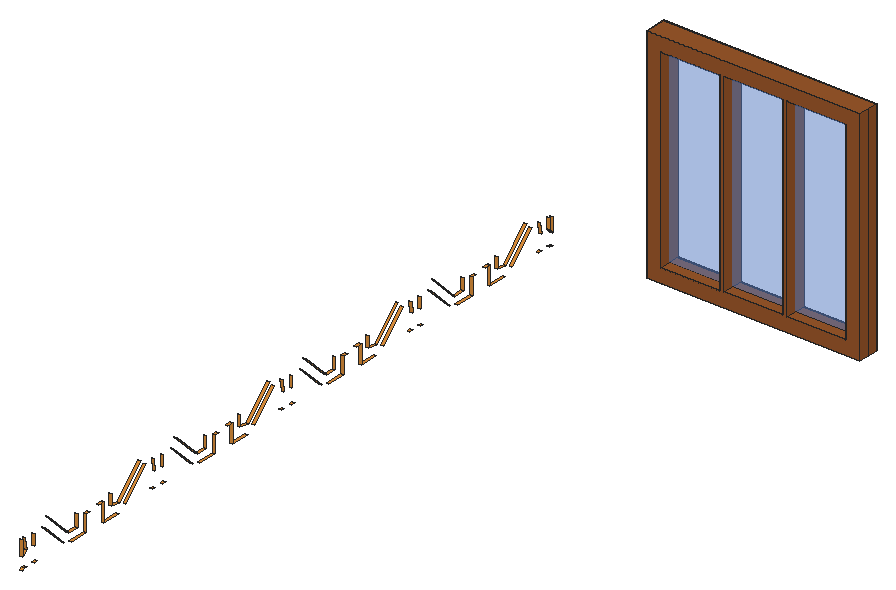
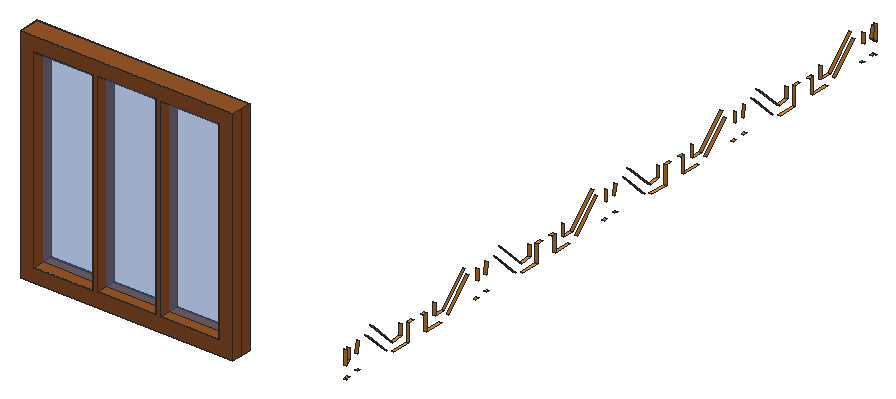
# SketchUp Ruby script. Lengths in inches.
U = 1.inch
M = Sketchup.active_model
def pt(a) = Geom::Point3d.new(a.map { |v| v * U })
def face(e, loops, mat)
  f = e.add_face(loops[0].map { |a| pt(a) })
  loops[1..].each { |l| e.add_face(l.map { |a| pt(a) }).erase! }
  f.material = f.back_material = mat if mat
  f
end
# faces: each face lists its corners as indices into pts; further lists are holes
def faces(e, pts, list, mat = nil) = list.each { |f| face(e, (f[0].is_a?(Array) ? f : [f]).map { |l| l.map { |i| pts[i] } }, mat) }
# xy, xz, yz: faces in a plane at the given z, y or x. An outline is a flat list of corners, or four numbers for a rectangle; further outlines are holes
def ring(l) = l.size == 4 ? [[l[0], l[1]], [l[2], l[1]], [l[2], l[3]], [l[0], l[3]]] : l.each_slice(2).to_a
def flat(e, list, mat, &to3) = list.each { |f| face(e, (f[0].is_a?(Array) ? f : [f]).map { |l| ring(l).map { |u, v| to3.(u, v) } }, mat) }
def xy(e, z, list, mat = nil) = flat(e, list, mat) { |x, y| [x, y, z] }
def xz(e, y, list, mat = nil) = flat(e, list, mat) { |x, z| [x, y, z] }
def yz(e, x, list, mat = nil) = flat(e, list, mat) { |y, z| [x, y, z] }
def lines(e, pts, list) = list.each { |a, b| e.add_line(pt(pts[a]), pt(pts[b])) }
# prism: a flat outline (further loops are holes) pulled along v
def prism(e, loops, v, mat = nil)
  f = face(e, loops, mat); d = Geom::Vector3d.new(v.map { |x| x * U })
  f.pushpull(f.normal.samedirection?(d) ? d.length : -d.length)
end
def box(e, o, s, mat = nil) = prism(e, [[o, [o[0] + s[0], o[1], o[2]], [o[0] + s[0], o[1] + s[1], o[2]], [o[0], o[1] + s[1], o[2]]]], [0, 0, s[2]], mat)
def at(x, y, z, deg = 0) = Geom::Transformation.translation(pt([x, y, z])) * Geom::Transformation.rotation(ORIGIN, Z_AXIS, deg.degrees)
def axes(o, x, y, z) = Geom::Transformation.new([*x, 0, *y, 0, *z, 0, *pt(o).to_a, 1])
def part(name) = M.definitions.add(name)
# library, detail: a bought-in or finely detailed component or shape, given as its bounding box
def library(name, o, s) = part(name).tap { |d| box(d.entities, o, s) }
def detail(e, o, s) = box(e.add_group.entities, o, s)
def put(e, d, t, mat = nil) = e.add_instance(d, t).tap { |i| i.material = mat if mat }
def group(e, t, mat = nil) = e.add_group.tap { |g| g.transformation = t; g.material = mat if mat }.entities
root = M.entities
M.materials.add("1056 AP 9903 Mellow Melon-N").color = [219, 142, 59]
M.materials.add("[Translucent Glass Blue]").color = [100, 149, 237]
M.materials["[Translucent Glass Blue]"].alpha = 0.5
M.materials.add("[Wood Cherry Original]").color = [152, 86, 42]
c1 = part("Group65\#3")
xy(c1.entities,0,[[-26.0625,-27.25,-9.48,27.25],[-8.29,-27.25,8.29,27.25],[9.48,-27.25,26.0625,27.25]])
c2 = part("Group64\#2")
prism(c2.entities,[[[30,-31.1875,0],[-30,-31.1875,0],[-30,31.1875,0],[30,31.1875,0]],[[-26.0625,27.25,0],[-26.0625,-27.25,0],[-9.48,-27.25,0],[-9.48,27.25,0]],[[26.0625,-27.25,0],[26.0625,27.25,0],[9.48,27.25,0],[9.48,-27.25,0]],[[8.29,-27.25,0],[8.29,27.25,0],[-8.29,27.25,0],[-8.29,-27.25,0]]],[0,0,5.875])
put(c2.entities,c1,at(0,0,2.9375),"[Translucent Glass Blue]")
xy(root,150.43,[[14.35,43.37,15.0625,48.53],[14.35,88.72,15.0625,93.87],[14.35,134.06,15.0625,139.21],[14.35,179.4,15.0625,184.56]],"1056 AP 9903 Mellow Melon-N")
xy(root,150.62,[[14.35,31.88,15.0625,37.08],[14.35,77.22,15.0625,82.42],[14.35,122.57,15.0625,127.77],[14.35,167.91,15.0625,173.11]],"1056 AP 9903 Mellow Melon-N")
xy(root,151.05,[[14.35,18.88,15.0625,19.75],[14.35,64.22,15.0625,65.1],[14.35,109.57,15.0625,110.44],[14.35,154.91,15.0625,155.79],[14.35,200.25,15.0625,201.13]],"1056 AP 9903 Mellow Melon-N")
xy(root,151.3,[[14.35,15.22,15.0625,16.07],[14.35,60.57,15.0625,61.42],[14.35,105.91,15.0625,106.76],[14.35,151.25,15.0625,152.1],[14.35,196.6,15.0625,197.45]],"1056 AP 9903 Mellow Melon-N")
xy(root,153.19,[[14.35,30.98,15.0625,34.05],[14.35,76.32,15.0625,79.39],[14.35,121.67,15.0625,124.73],[14.35,167.01,15.0625,170.08]],"1056 AP 9903 Mellow Melon-N")
xy(root,155.34,[[14.35,37.08,15.0625,38.38],[14.35,82.42,15.0625,83.72],[14.35,127.77,15.0625,129.07],[14.35,173.11,15.0625,174.41]],"1056 AP 9903 Mellow Melon-N")
xy(root,155.63,[[14.35,41.65,15.0625,43.37],[14.35,87,15.0625,88.72],[14.35,132.34,15.0625,134.06],[14.35,177.68,15.0625,179.4]],"1056 AP 9903 Mellow Melon-N")
xz(root,14.79,[[14.35,154.31,15.0625,158.67]],"1056 AP 9903 Mellow Melon-N")
xz(root,18.88,[[14.35,155.375,15.0625,158.35]],"1056 AP 9903 Mellow Melon-N")
xz(root,34.05,[[14.35,153.19,15.0625,156.6]],"1056 AP 9903 Mellow Melon-N")
xz(root,37.08,[[14.35,150.62,15.0625,155.34]],"1056 AP 9903 Mellow Melon-N")
xz(root,43.37,[[14.35,150.43,15.0625,155.63]],"1056 AP 9903 Mellow Melon-N")
xz(root,45.95,[[14.35,153.47,15.0625,156.53]],"1056 AP 9903 Mellow Melon-N")
xz(root,64.22,[[14.35,155.375,15.0625,158.35]],"1056 AP 9903 Mellow Melon-N")
xz(root,79.39,[[14.35,153.19,15.0625,156.6]],"1056 AP 9903 Mellow Melon-N")
xz(root,82.42,[[14.35,150.62,15.0625,155.34]],"1056 AP 9903 Mellow Melon-N")
xz(root,88.72,[[14.35,150.43,15.0625,155.63]],"1056 AP 9903 Mellow Melon-N")
xz(root,91.29,[[14.35,153.47,15.0625,156.53]],"1056 AP 9903 Mellow Melon-N")
xz(root,109.57,[[14.35,155.375,15.0625,158.35]],"1056 AP 9903 Mellow Melon-N")
xz(root,124.73,[[14.35,153.19,15.0625,156.6]],"1056 AP 9903 Mellow Melon-N")
xz(root,127.77,[[14.35,150.62,15.0625,155.34]],"1056 AP 9903 Mellow Melon-N")
xz(root,134.06,[[14.35,150.43,15.0625,155.63]],"1056 AP 9903 Mellow Melon-N")
xz(root,136.64,[[14.35,153.47,15.0625,156.53]],"1056 AP 9903 Mellow Melon-N")
xz(root,154.91,[[14.35,155.375,15.0625,158.35]],"1056 AP 9903 Mellow Melon-N")
xz(root,170.08,[[14.35,153.19,15.0625,156.6]],"1056 AP 9903 Mellow Melon-N")
xz(root,173.11,[[14.35,150.62,15.0625,155.34]],"1056 AP 9903 Mellow Melon-N")
xz(root,179.4,[[14.35,150.43,15.0625,155.63]],"1056 AP 9903 Mellow Melon-N")
xz(root,181.98,[[14.35,153.47,15.0625,156.53]],"1056 AP 9903 Mellow Melon-N")
xz(root,200.25,[[14.35,155.375,15.0625,158.35]],"1056 AP 9903 Mellow Melon-N")
xz(root,201.3125,[[14.35,154.31,15.0625,158.35]],"1056 AP 9903 Mellow Melon-N")
p = [[15.0625,15.22,151.3],[15.0625,14.79,150.86],[14.35,14.79,150.86],[14.35,15.22,151.3],[15.0625,201.3125,150.86],[15.0625,201.13,151.05],
  [14.35,201.13,151.05],[14.35,201.3125,150.86],[15.0625,29.28,151.45],[15.0625,22.375,158.35],[14.35,22.375,158.35],[14.35,29.28,151.45],
  [15.0625,74.625,151.45],[15.0625,67.72,158.35],[14.35,67.72,158.35],[14.35,74.625,151.45],[15.0625,119.97,151.45],[15.0625,113.0625,158.35],
  [14.35,113.0625,158.35],[14.35,119.97,151.45],[15.0625,165.3125,151.45],[15.0625,158.41,158.35],[14.35,158.41,158.35],[14.35,165.3125,151.45],
  [15.0625,58.01,158.67],[15.0625,51.11,151.76],[14.35,51.11,151.76],[14.35,58.01,158.67],[15.0625,103.35,158.67],[15.0625,96.45,151.76],
  [14.35,96.45,151.76],[14.35,103.35,158.67],[15.0625,148.7,158.67],[15.0625,141.79,151.76],[14.35,141.79,151.76],[14.35,148.7,158.67],
  [15.0625,194.04,158.67],[15.0625,187.14,151.76],[14.35,187.14,151.76],[14.35,194.04,158.67],[15.0625,45.95,153.47],[15.0625,48.93,153.04],
  [14.35,48.93,153.04],[14.35,45.95,153.47],[15.0625,56.26,160.37],[14.35,56.26,160.37],[15.0625,91.29,153.47],[15.0625,94.27,153.04],
  [14.35,94.27,153.04],[14.35,91.29,153.47],[15.0625,101.6,160.37],[14.35,101.6,160.37],[15.0625,136.64,153.47],[15.0625,139.62,153.04],
  [14.35,139.62,153.04],[14.35,136.64,153.47],[15.0625,146.95,160.37],[14.35,146.95,160.37],[15.0625,181.98,153.47],[15.0625,184.96,153.04],
  [14.35,184.96,153.04],[14.35,181.98,153.47],[15.0625,192.29,160.37],[14.35,192.29,160.37],[15.0625,23.65,160.53],[15.0625,30.98,153.19],
  [14.35,30.98,153.19],[14.35,23.65,160.53],[15.0625,68.99,160.53],[15.0625,76.32,153.19],[14.35,76.32,153.19],[14.35,68.99,160.53],
  [15.0625,114.34,160.53],[15.0625,121.67,153.19],[14.35,121.67,153.19],[14.35,114.34,160.53],[15.0625,159.68,160.53],[15.0625,167.01,153.19],
  [14.35,167.01,153.19],[14.35,159.68,160.53],[15.0625,14.79,154.31],[15.0625,16.08,155.61],[14.35,16.08,155.61],[14.35,14.79,154.31],
  [15.0625,200.25,155.375],[15.0625,201.3125,154.31],[14.35,201.3125,154.31],[14.35,200.25,155.375],[15.0625,15.64,158.67],[14.35,15.64,158.67],
  [15.0625,61.42,155.61],[15.0625,60.99,158.67],[14.35,60.99,158.67],[14.35,61.42,155.61],[15.0625,106.76,155.61],[15.0625,106.33,158.67],
  [14.35,106.33,158.67],[14.35,106.76,155.61],[15.0625,152.11,155.61],[15.0625,151.67,158.67],[14.35,151.67,158.67],[14.35,152.11,155.61],
  [15.0625,197.45,155.61],[15.0625,197.02,158.67],[14.35,197.02,158.67],[14.35,197.45,155.61],[39.5625,206.8125,150.375],[39.5625,206.8125,212.75],
  [99.5625,206.8125,212.75],[99.5625,206.8125,150.375]]
faces(root,p,[[0,1,2,3],[4,5,6,7],[8,9,10,11],[12,13,14,15],[16,17,18,19],[20,21,22,23],[24,25,26,27],[28,29,30,31],
  [32,33,34,35],[36,37,38,39],[40,41,42,43],[41,44,45,42],[46,47,48,49],[47,50,51,48],[52,53,54,55],[53,56,57,54],
  [58,59,60,61],[59,62,63,60],[64,65,66,67],[68,69,70,71],[72,73,74,75],[76,77,78,79],[80,81,82,83],[84,85,86,87],
  [81,88,89,82],[90,91,92,93],[94,95,96,97],[98,99,100,101],[102,103,104,105]],"1056 AP 9903 Mellow Melon-N")
lines(root,p,[[106,107],[108,109],[109,106]])
put(root,c2,axes([69.5625,209.75,181.5625],[1,0,0],[0,0,1],[0,-1,0]),"[Wood Cherry Original]")
